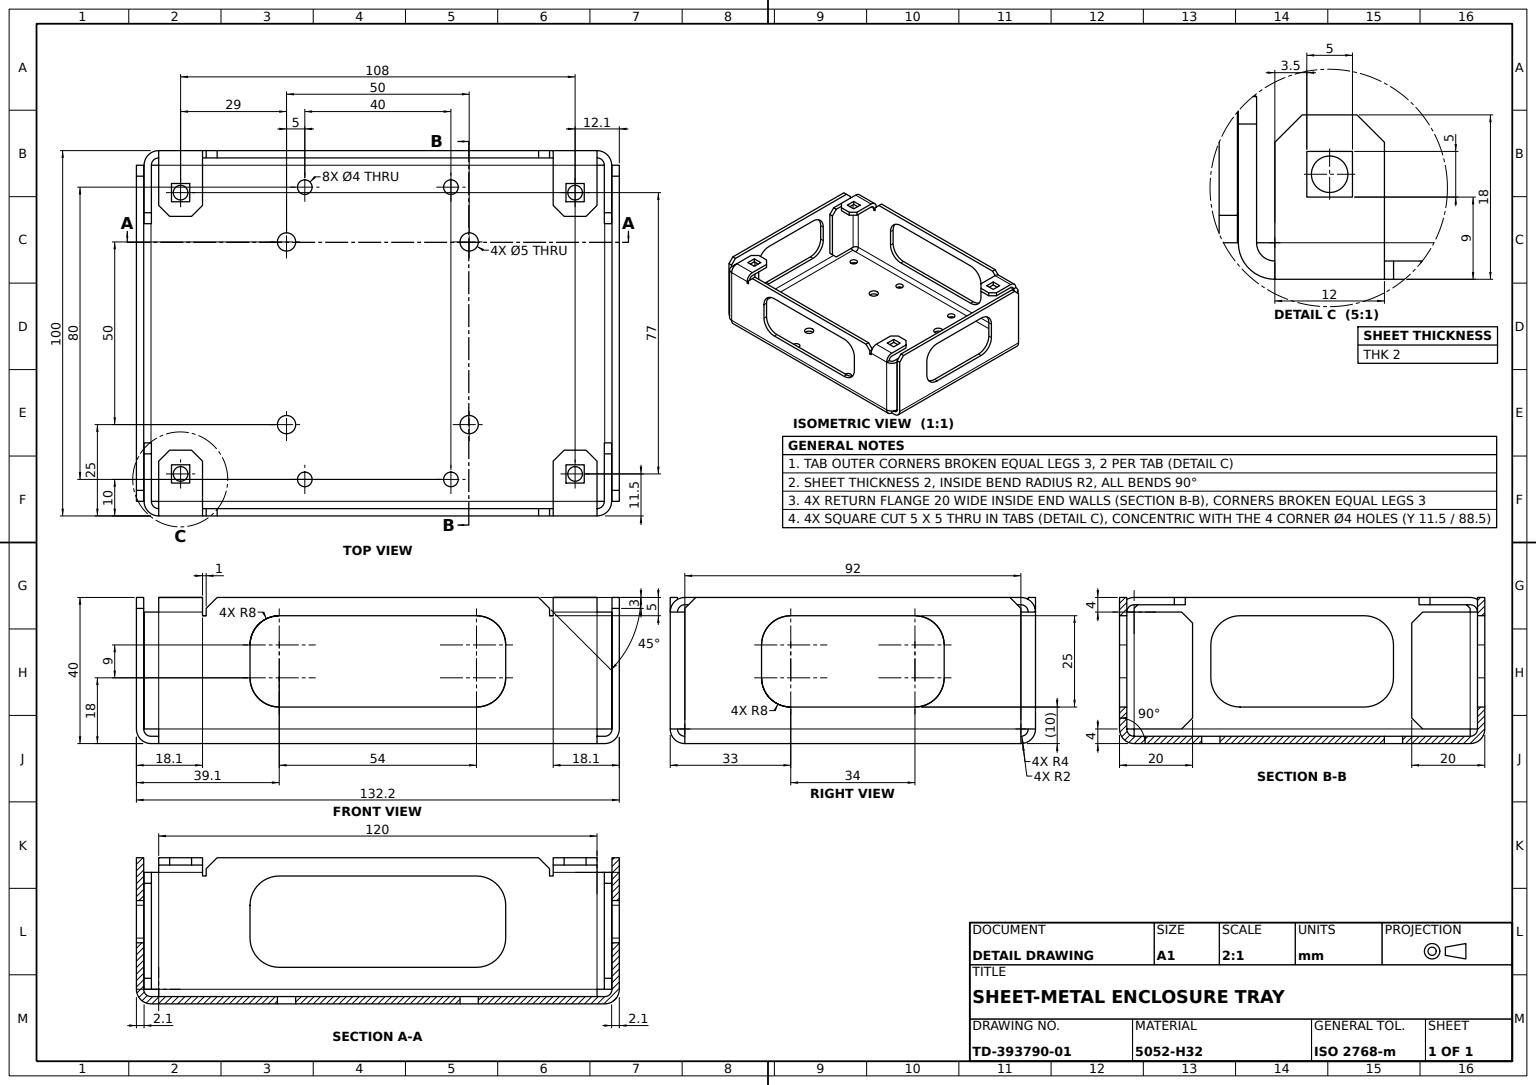
solid
v1 (-27,10,-48)
v2 (27,10,-48)
e1 v1 v2 LINE
v3 (27,10,-50)
e2 v2 v3 LINE
v4 (-27,10,-50)
e3 v4 v3 LINE
e4 v1 v4 LINE
face PLANE(AX(P(-27,10,-48),D(0,1,0),D(0,0,1))) [e1 e2 -e3 -e4]
v5 (-35,27,-48)
v6 (-35,18,-48)
e5 v5 v6 LINE
v7 (-35,18,-50)
e6 v6 v7 LINE
v8 (-35,27,-50)
e7 v8 v7 LINE
e8 v5 v8 LINE
face PLANE(AX(P(-35,18,-48),D(1,0,0),D(0,1,0))) [e5 e6 -e7 -e8]
v9 (47,37,-50)
v10 (47,37,-48)
e9 v9 v10 LINE
v11 (44,40,-50)
e10 v11 v9 LINE
v12 (44,40,-48)
e11 v12 v11 LINE
e12 v10 v12 LINE
face PLANE(AX(P(44,40,-50),D(0.707106781,0.707106781,0),D(0,0,1))) [-e9 -e10 -e11 -e12]
v13 (60,38,46)
v14 (60,36,48)
e13 v13 v14 CIRCLE(AX(P(60,36,46),D(1,0,0),D(0,0,-1)),2)
v15 (60,40,46)
e14 v13 v15 LINE
v16 (60,36,50)
e15 v15 v16 CIRCLE(AX(P(60,36,46),D(1,0,0),D(0,0,-1)),4)
e16 v14 v16 LINE
face PLANE(AX(P(60,36,46),D(-1,0,0),D(0,0,1))) rev [-e13 e14 e15 -e16]
v17 (64.1,18,25)
v18 (66.1,18,25)
e17 v17 v18 LINE
v19 (66.1,10,17)
e18 v18 v19 CIRCLE(AX(P(66.1,18,17),D(1,0,0),D(0,-1,0)),8)
v20 (64.1,10,17)
e19 v20 v19 LINE
e20 v17 v20 CIRCLE(AX(P(64.1,18,17),D(1,0,0),D(0,-1,0)),8)
face CYL(AX(P(64.1,18,17),D(1,0,0),D(0,1,0)),8) rev [e17 e18 -e19 -e20]
v21 (64.1,35,-17)
v22 (66.1,35,-17)
e21 v21 v22 LINE
v23 (64.1,27,-25)
e22 v23 v21 CIRCLE(AX(P(64.1,27,-17),D(1,0,0),D(0,-1,0)),8)
v24 (66.1,27,-25)
e23 v23 v24 LINE
e24 v24 v22 CIRCLE(AX(P(66.1,27,-17),D(1,0,0),D(0,-1,0)),8)
face CYL(AX(P(64.1,27,-17),D(1,0,0),D(0,1,0)),8) rev [-e21 -e22 e23 e24]
v25 (48,38,46)
e25 v25 v13 LINE
v26 (48,38,35)
e26 v26 v25 LINE
v27 (51,38,32)
e27 v26 v27 LINE
v28 (57,38,32)
e28 v28 v27 LINE
v29 (60,38,35)
e29 v28 v29 LINE
e30 v13 v29 LINE
v30 (56.5,38,41)
v31 (56.5,38,36)
e31 v30 v31 LINE
v32 (51.5,38,36)
e32 v31 v32 LINE
v33 (51.5,38,41)
e33 v32 v33 LINE
e34 v33 v30 LINE
face PLANE(AX(P(0,38,0),D(0,-1,0),D(0,0,-1))) [-e25 -e26 e27 -e28 e29 -e30] [e31 e32 e33 e34]
v34 (27,35,-48)
v35 (-27,35,-48)
e35 v34 v35 LINE
v36 (35,27,-48)
e36 v36 v34 CIRCLE(AX(P(27,27,-48),D(0,0,1),D(-1,0,0)),8)
v37 (35,18,-48)
e37 v37 v36 LINE
e38 v2 v37 CIRCLE(AX(P(27,18,-48),D(0,0,1),D(1,0,0)),8)
e39 v6 v1 CIRCLE(AX(P(-27,18,-48),D(0,0,1),D(-1,0,0)),8)
e40 v35 v5 CIRCLE(AX(P(-27,27,-48),D(0,0,1),D(-1,0,0)),8)
v38 (-47,35,-48)
v39 (-47,37,-48)
e41 v38 v39 LINE
v40 (-48,35,-48)
e42 v40 v38 LINE
v41 (-48,36,-48)
e43 v41 v40 LINE
v42 (-60,36,-48)
e44 v42 v41 LINE
v43 (-60,4,-48)
e45 v43 v42 LINE
v44 (60,4,-48)
e46 v44 v43 LINE
v45 (60,36,-48)
e47 v45 v44 LINE
v46 (48,36,-48)
e48 v46 v45 LINE
v47 (48,35,-48)
e49 v47 v46 LINE
v48 (47,35,-48)
e50 v48 v47 LINE
e51 v10 v48 LINE
v49 (-44,40,-48)
e52 v49 v12 LINE
e53 v49 v39 LINE
face PLANE(AX(P(0,0,-48),D(0,0,1),D(0,-1,0))) [-e35 -e36 -e37 -e38 -e1 -e39 -e5 -e40] [-e41 -e42 -e43 -e44 -e45 -e46 -e47 -e48 -e49 -e50 -e51 e12 -e52 e53]
v50 (51.5,40,36)
e54 v32 v50 LINE
v51 (56.5,40,36)
e55 v31 v51 LINE
e56 v51 v50 LINE
face PLANE(AX(P(56.5,38,36),D(0,0,-1),D(0,1,0))) rev [-e54 -e32 e55 e56]
v52 (-47,37,-50)
e57 v39 v52 LINE
v53 (-44,40,-50)
e58 v53 v49 LINE
e59 v52 v53 LINE
face PLANE(AX(P(-47,37,-48),D(-0.707106781,0.707106781,0),D(0,0,1))) [-e57 -e53 -e58 -e59]
v54 (-48,36,-50)
e60 v41 v54 LINE
v55 (-48,35,-50)
e61 v40 v55 LINE
e62 v55 v54 LINE
face PLANE(AX(P(-48,36,-48),D(1,0,0),D(0,0,-1))) [-e60 e43 e61 e62]
v56 (-51.5,38,36)
v57 (-51.5,40,36)
e63 v56 v57 LINE
v58 (-56.5,40,36)
e64 v58 v57 LINE
v59 (-56.5,38,36)
e65 v59 v58 LINE
e66 v59 v56 LINE
face PLANE(AX(P(-56.5,38,36),D(0,0,1),D(0,-1,0))) [e63 -e64 -e65 e66]
v60 (44,40,48)
v61 (47,37,48)
e67 v60 v61 LINE
v62 (44,40,50)
e68 v62 v60 LINE
v63 (47,37,50)
e69 v63 v62 LINE
e70 v61 v63 LINE
face PLANE(AX(P(47,37,48),D(0.707106781,0.707106781,0),D(0,0,-1))) [-e67 -e68 -e69 -e70]
v64 (-62,4,-33)
v65 (-62,4,-46)
e71 v64 v65 LINE
v66 (-62,36,-46)
e72 v66 v65 LINE
v67 (-62,36,-33)
e73 v66 v67 LINE
v68 (-62,33,-30)
e74 v67 v68 LINE
v69 (-62,7,-30)
e75 v68 v69 LINE
e76 v69 v64 LINE
face PLANE(AX(P(-62,0,0),D(1,0,0),D(0,0,-1))) [e71 -e72 e73 e74 e75 e76]
v70 (48,36,-50)
v71 (60,36,-50)
e77 v70 v71 LINE
v72 (48,40,-46)
e78 v72 v70 CIRCLE(AX(P(48,36,-46),D(-1,0,0),D(0,0,1)),4)
v73 (60,40,-46)
e79 v72 v73 LINE
e80 v71 v73 CIRCLE(AX(P(60,36,-46),D(1,0,0),D(0,0,1)),4)
face CYL(AX(P(48,36,-46),D(-1,0,0),D(0,1,0)),4) [-e77 -e78 e79 -e80]
v74 (25,0,-27.5)
v75 (25,2,-27.5)
e81 v74 v75 LINE
v76 (25,0,-22.5)
e82 v76 v74 CIRCLE(AX(P(25,0,-25),D(0,1,0),D(0,0,1)),2.5)
v77 (25,2,-22.5)
e83 v76 v77 LINE
e84 v77 v75 CIRCLE(AX(P(25,2,-25),D(0,1,0),D(0,0,1)),2.5)
face CYL(AX(P(25,0,-25),D(0,1,0),D(0,0,1)),2.5) rev [-e81 -e82 e83 e84]
v78 (-60,4,-50)
v79 (-60,36,-50)
e85 v78 v79 LINE
v80 (-64,4,-46)
e86 v80 v78 CIRCLE(AX(P(-60,4,-46),D(0,-1,0),D(0,0,-1)),4)
v81 (-64,36,-46)
e87 v80 v81 LINE
e88 v79 v81 CIRCLE(AX(P(-60,36,-46),D(0,1,0),D(0,0,-1)),4)
face CYL(AX(P(-60,4,-46),D(0,-1,0),D(-1,0,0)),4) [-e85 -e86 e87 -e88]
v82 (60,2,46)
v83 (60,0,46)
e89 v82 v83 LINE
v84 (62.1,0,46)
e90 v84 v83 LINE
v85 (62.1,2,46)
e91 v85 v84 LINE
e92 v85 v82 LINE
face PLANE(AX(P(62.1,2,46),D(0,0,-1),D(0,-1,0))) rev [e89 -e90 -e91 e92]
v86 (62,7,-30)
v87 (62,33,-30)
e93 v86 v87 LINE
v88 (64,7,-30)
e94 v86 v88 LINE
v89 (64,33,-30)
e95 v88 v89 LINE
e96 v89 v87 LINE
face PLANE(AX(P(64,4,-30),D(0,0,1),D(1,0,0))) [-e93 e94 e95 e96]
v90 (64.1,18,-25)
e97 v90 v23 LINE
v91 (64.1,35,17)
e98 v21 v91 LINE
v92 (64.1,27,25)
e99 v91 v92 CIRCLE(AX(P(64.1,27,17),D(1,0,0),D(0,-1,0)),8)
e100 v92 v17 LINE
v93 (64.1,10,-17)
e101 v20 v93 LINE
e102 v93 v90 CIRCLE(AX(P(64.1,18,-17),D(1,0,0),D(0,1,0)),8)
v94 (64.1,4,46)
v95 (64.1,4,-46)
e103 v94 v95 LINE
v96 (64.1,37,46)
e104 v96 v94 LINE
v97 (64.1,40,43)
e105 v96 v97 LINE
v98 (64.1,40,-43)
e106 v98 v97 LINE
v99 (64.1,37,-46)
e107 v98 v99 LINE
e108 v95 v99 LINE
face PLANE(AX(P(64.1,0,0),D(-1,0,0),D(0,-1,0))) [e97 e22 e98 e99 e100 e20 e101 e102] [-e103 -e104 e105 -e106 e107 -e108]
v100 (54,0,36.5)
v101 (54,2,36.5)
e109 v100 v101 LINE
v102 (54,2,40.5)
e110 v101 v102 CIRCLE(AX(P(54,2,38.5),D(0,1,0),D(0,0,1)),2)
v103 (54,0,40.5)
e111 v103 v102 LINE
e112 v100 v103 CIRCLE(AX(P(54,0,38.5),D(0,1,0),D(0,0,1)),2)
face CYL(AX(P(54,0,38.5),D(0,1,0),D(0,0,1)),2) rev [e109 e110 -e111 -e112]
v104 (-51.5,40,41)
v105 (-56.5,40,41)
e113 v104 v105 LINE
v106 (-51.5,38,41)
e114 v106 v104 LINE
v107 (-56.5,38,41)
e115 v106 v107 LINE
e116 v107 v105 LINE
face PLANE(AX(P(-56.5,38,41),D(0,0,-1),D(0,1,0))) [-e113 -e114 e115 e116]
v108 (47,35,50)
e117 v63 v108 LINE
v109 (47,35,48)
e118 v109 v108 LINE
e119 v109 v61 LINE
face PLANE(AX(P(47,35,48),D(1,0,0),D(0,0,-1))) [e117 -e118 e119 e70]
v110 (-64.1,35,17)
v111 (-64.1,27,25)
e120 v110 v111 CIRCLE(AX(P(-64.1,27,17),D(1,0,0),D(0,-1,0)),8)
v112 (-66.1,27,25)
e121 v111 v112 LINE
v113 (-66.1,35,17)
e122 v113 v112 CIRCLE(AX(P(-66.1,27,17),D(1,0,0),D(0,-1,0)),8)
e123 v110 v113 LINE
face CYL(AX(P(-64.1,27,17),D(-1,0,0),D(0,-1,0)),8) rev [e120 e121 -e122 -e123]
v114 (-35,18,48)
v115 (-35,18,50)
e124 v114 v115 LINE
v116 (-27,10,50)
e125 v115 v116 CIRCLE(AX(P(-27,18,50),D(0,0,1),D(-1,0,0)),8)
v117 (-27,10,48)
e126 v117 v116 LINE
e127 v114 v117 CIRCLE(AX(P(-27,18,48),D(0,0,1),D(-1,0,0)),8)
face CYL(AX(P(-27,18,48),D(0,0,1),D(1,0,0)),8) rev [e124 e125 -e126 -e127]
v118 (-54,2,-40.5)
v119 (-54,2,-36.5)
e128 v118 v119 CIRCLE(AX(P(-54,2,-38.5),D(0,1,0),D(0,0,1)),2)
v120 (-54,0,-36.5)
e129 v120 v119 LINE
v121 (-54,0,-40.5)
e130 v121 v120 CIRCLE(AX(P(-54,0,-38.5),D(0,1,0),D(0,0,1)),2)
e131 v121 v118 LINE
face CYL(AX(P(-54,0,-38.5),D(0,1,0),D(0,0,1)),2) rev [e128 -e129 -e130 e131]
v122 (-64.1,18,-25)
v123 (-64.1,27,-25)
e132 v122 v123 LINE
v124 (-66.1,27,-25)
e133 v123 v124 LINE
v125 (-66.1,18,-25)
e134 v125 v124 LINE
e135 v122 v125 LINE
face PLANE(AX(P(-64.1,18,-25),D(0,0,1),D(1,0,0))) [e132 e133 -e134 -e135]
v126 (35,27,-50)
v127 (27,35,-50)
e136 v126 v127 CIRCLE(AX(P(27,27,-50),D(0,0,1),D(-1,0,0)),8)
v128 (-27,35,-50)
e137 v127 v128 LINE
e138 v128 v8 CIRCLE(AX(P(-27,27,-50),D(0,0,1),D(-1,0,0)),8)
e139 v7 v4 CIRCLE(AX(P(-27,18,-50),D(0,0,1),D(-1,0,0)),8)
v129 (35,18,-50)
e140 v3 v129 CIRCLE(AX(P(27,18,-50),D(0,0,1),D(1,0,0)),8)
e141 v129 v126 LINE
v130 (-47,35,-50)
e142 v52 v130 LINE
e143 v53 v11 LINE
v131 (47,35,-50)
e144 v131 v9 LINE
v132 (48,35,-50)
e145 v132 v131 LINE
e146 v70 v132 LINE
v133 (60,4,-50)
e147 v71 v133 LINE
e148 v78 v133 LINE
e149 v79 v54 LINE
e150 v130 v55 LINE
face PLANE(AX(P(0,0,-50),D(0,0,1),D(0,-1,0))) rev [e136 e137 e138 e7 e139 e3 e140 e141] [-e142 e59 e143 e10 -e144 -e145 -e146 e77 e147 -e148 e85 e149 -e62 -e150]
face PLANE(AX(P(60,40,-50),D(0,-1,0),D(0,0,-1))) rev [e52 e11 -e143 e58]
v134 (66.1,35,17)
e151 v22 v134 LINE
e152 v91 v134 LINE
face PLANE(AX(P(64.1,35,17),D(0,1,0),D(-1,0,0))) rev [e21 e151 -e152 -e98]
v135 (-44,40,50)
e153 v62 v135 LINE
v136 (-47,37,50)
e154 v135 v136 LINE
v137 (-47,35,50)
e155 v137 v136 LINE
v138 (-48,35,50)
e156 v138 v137 LINE
v139 (-48,36,50)
e157 v139 v138 LINE
v140 (-60,36,50)
e158 v139 v140 LINE
v141 (-60,4,50)
e159 v140 v141 LINE
v142 (60,4,50)
e160 v142 v141 LINE
e161 v142 v16 LINE
v143 (48,36,50)
e162 v16 v143 LINE
v144 (48,35,50)
e163 v144 v143 LINE
e164 v108 v144 LINE
v145 (35,18,50)
v146 (35,27,50)
e165 v145 v146 LINE
v147 (27,10,50)
e166 v147 v145 CIRCLE(AX(P(27,18,50),D(0,0,1),D(1,0,0)),8)
e167 v116 v147 LINE
v148 (-35,27,50)
e168 v148 v115 LINE
v149 (-27,35,50)
e169 v149 v148 CIRCLE(AX(P(-27,27,50),D(0,0,1),D(-1,0,0)),8)
v150 (27,35,50)
e170 v150 v149 LINE
e171 v146 v150 CIRCLE(AX(P(27,27,50),D(0,0,1),D(-1,0,0)),8)
face PLANE(AX(P(0,0,50),D(0,0,-1),D(-1,0,0))) rev [e69 e153 e154 -e155 -e156 -e157 e158 e159 -e160 e161 e162 -e163 -e164 -e117] [-e165 -e166 -e167 -e125 -e168 -e169 -e170 -e171]
v151 (-48,38,-46)
v152 (-48,40,-46)
e172 v151 v152 LINE
v153 (-48,40,-35)
e173 v153 v152 LINE
v154 (-48,38,-35)
e174 v153 v154 LINE
e175 v154 v151 LINE
face PLANE(AX(P(-48,40,-48),D(-1,0,0),D(0,0,1))) rev [e172 -e173 e174 e175]
v155 (48,36,48)
e176 v14 v155 LINE
e177 v155 v25 CIRCLE(AX(P(48,36,46),D(-1,0,0),D(0,0,-1)),2)
face CYL(AX(P(60,36,46),D(1,0,0),D(0,1,0)),2) rev [e176 e177 e25 e13]
v156 (54,0,-36.5)
v157 (54,0,-40.5)
e178 v156 v157 CIRCLE(AX(P(54,0,-38.5),D(0,1,0),D(0,0,1)),2)
v158 (54,2,-36.5)
e179 v156 v158 LINE
v159 (54,2,-40.5)
e180 v158 v159 CIRCLE(AX(P(54,2,-38.5),D(0,1,0),D(0,0,1)),2)
e181 v157 v159 LINE
face CYL(AX(P(54,0,-38.5),D(0,1,0),D(0,0,1)),2) rev [-e178 e179 e180 -e181]
v160 (-64,4,-33)
e182 v160 v80 LINE
e183 v65 v80 LINE
e184 v64 v160 LINE
face PLANE(AX(P(-64,4,-30),D(0,-1,0),D(0,0,-1))) [e182 -e183 -e71 e184]
v161 (-60,40,-46)
e185 v161 v79 CIRCLE(AX(P(-60,36,-46),D(-1,0,0),D(0,0,1)),4)
e186 v161 v152 LINE
e187 v54 v152 CIRCLE(AX(P(-48,36,-46),D(1,0,0),D(0,0,1)),4)
face CYL(AX(P(-60,36,-46),D(-1,0,0),D(0,1,0)),4) [-e185 e186 -e187 -e149]
v162 (-57,40,-32)
v163 (-51,40,-32)
e188 v162 v163 LINE
e189 v163 v153 LINE
v164 (-60,40,-35)
e190 v161 v164 LINE
e191 v164 v162 LINE
v165 (-51.5,40,-41)
v166 (-56.5,40,-41)
e192 v165 v166 LINE
v167 (-51.5,40,-36)
e193 v167 v165 LINE
v168 (-56.5,40,-36)
e194 v168 v167 LINE
e195 v166 v168 LINE
face PLANE(AX(P(0,40,0),D(0,-1,0),D(0,0,1))) rev [e188 e189 e173 -e186 e190 e191] [-e192 -e193 -e194 -e195]
v169 (60,40,-35)
v170 (60,38,-35)
e196 v169 v170 LINE
v171 (57,40,-32)
e197 v171 v169 LINE
v172 (57,38,-32)
e198 v172 v171 LINE
e199 v170 v172 LINE
face PLANE(AX(P(60,40,-35),D(-0.707106781,0,-0.707106781),D(0,-1,0))) rev [-e196 -e197 -e198 -e199]
v173 (57,40,32)
e200 v173 v28 LINE
v174 (51,40,32)
e201 v27 v174 LINE
e202 v173 v174 LINE
face PLANE(AX(P(48,40,32),D(0,0,1),D(0,-1,0))) rev [e200 e28 e201 -e202]
v175 (-48,40,35)
v176 (-48,40,46)
e203 v175 v176 LINE
v177 (-48,38,46)
e204 v177 v176 LINE
v178 (-48,38,35)
e205 v178 v177 LINE
e206 v178 v175 LINE
face PLANE(AX(P(-48,40,48),D(1,0,0),D(0,0,-1))) [e203 -e204 -e205 e206]
v179 (20,0,38)
v180 (20,2,38)
e207 v179 v180 LINE
v181 (20,0,42)
e208 v181 v179 CIRCLE(AX(P(20,0,40),D(0,1,0),D(0,0,1)),2)
v182 (20,2,42)
e209 v181 v182 LINE
e210 v182 v180 CIRCLE(AX(P(20,2,40),D(0,1,0),D(0,0,1)),2)
face CYL(AX(P(20,0,40),D(0,1,0),D(0,0,1)),2) rev [-e207 -e208 e209 e210]
v183 (-64,4,46)
e211 v141 v183 CIRCLE(AX(P(-60,4,46),D(0,-1,0),D(0,0,1)),4)
v184 (-64,36,46)
e212 v184 v140 CIRCLE(AX(P(-60,36,46),D(0,1,0),D(0,0,1)),4)
e213 v184 v183 LINE
face CYL(AX(P(-60,36,46),D(0,1,0),D(-1,0,0)),4) [-e211 -e159 -e212 e213]
v185 (-56.5,38,-41)
e214 v185 v166 LINE
v186 (-51.5,38,-41)
e215 v186 v185 LINE
e216 v186 v165 LINE
face PLANE(AX(P(-56.5,38,-41),D(0,0,-1),D(0,1,0))) rev [e192 -e214 -e215 e216]
v187 (-64,7,-30)
e217 v187 v69 LINE
e218 v160 v187 LINE
face PLANE(AX(P(-64,7,-30),D(0,0.707106781,-0.707106781),D(1,0,0))) rev [-e217 -e218 -e184 -e76]
v188 (62.1,2,-46)
v189 (62.1,0,-46)
e219 v188 v189 LINE
v190 (60,0,-46)
e220 v189 v190 LINE
v191 (60,2,-46)
e221 v191 v190 LINE
e222 v188 v191 LINE
face PLANE(AX(P(62.1,2,-46),D(0,0,-1),D(0,-1,0))) [e219 e220 -e221 -e222]
v192 (60,40,35)
e223 v29 v192 LINE
e224 v192 v173 LINE
face PLANE(AX(P(57,40,32),D(-0.707106781,0,0.707106781),D(0,-1,0))) rev [-e223 -e29 -e200 -e224]
v193 (-47,35,48)
e225 v193 v137 LINE
v194 (-47,37,48)
e226 v136 v194 LINE
e227 v194 v193 LINE
face PLANE(AX(P(-47,40,48),D(-1,0,0),D(0,0,1))) [e225 e155 e226 e227]
v195 (-57,38,-32)
v196 (-60,38,-35)
e228 v195 v196 LINE
e229 v162 v195 LINE
e230 v196 v164 LINE
face PLANE(AX(P(-57,40,-32),D(0.707106781,0,-0.707106781),D(0,-1,0))) rev [-e228 -e229 -e191 -e230]
v197 (62,36,-33)
v198 (62,36,-46)
e231 v197 v198 LINE
v199 (64,36,-33)
e232 v197 v199 LINE
v200 (64,36,-46)
e233 v199 v200 LINE
e234 v198 v200 LINE
face PLANE(AX(P(64,36,-30),D(0,1,0),D(0,0,1))) [-e231 e232 e233 -e234]
v201 (-48,35,48)
e235 v201 v138 LINE
v202 (-48,36,48)
e236 v201 v202 LINE
e237 v202 v139 LINE
face PLANE(AX(P(-48,35,48),D(1,0,0),D(0,0,-1))) [e157 -e235 e236 e237]
v203 (66.1,40,43)
e238 v97 v203 LINE
v204 (66.1,37,46)
e239 v204 v96 LINE
e240 v203 v204 LINE
face PLANE(AX(P(66.1,37,46),D(0,-0.707106781,-0.707106781),D(-1,0,0))) rev [-e238 -e105 -e239 -e240]
v205 (56.5,40,41)
e241 v30 v205 LINE
e242 v205 v51 LINE
face PLANE(AX(P(56.5,38,36),D(1,0,0),D(0,0,-1))) rev [e241 e242 -e55 -e31]
e243 v66 v81 LINE
v206 (-64,36,-33)
e244 v81 v206 LINE
e245 v206 v67 LINE
face PLANE(AX(P(-64,36,-48),D(0,1,0),D(0,0,1))) [-e73 e243 e244 e245]
v207 (-51,38,-32)
e246 v195 v207 LINE
e247 v207 v163 LINE
face PLANE(AX(P(-48,40,-32),D(0,0,-1),D(0,1,0))) rev [e246 e247 -e188 e229]
v208 (-60,40,46)
e248 v176 v208 LINE
e249 v140 v208 CIRCLE(AX(P(-60,36,46),D(-1,0,0),D(0,0,-1)),4)
e250 v176 v139 CIRCLE(AX(P(-48,36,46),D(1,0,0),D(0,0,-1)),4)
face CYL(AX(P(-48,36,46),D(1,0,0),D(0,1,0)),4) [e248 -e249 -e158 -e250]
v209 (-51.5,38,-36)
e251 v209 v186 LINE
e252 v209 v167 LINE
face PLANE(AX(P(-51.5,38,-36),D(1,0,0),D(0,0,-1))) rev [-e216 -e251 e252 e193]
v210 (-60,38,46)
e253 v210 v208 LINE
v211 (-60,36,48)
e254 v211 v210 CIRCLE(AX(P(-60,36,46),D(-1,0,0),D(0,0,-1)),2)
e255 v211 v140 LINE
face PLANE(AX(P(-60,36,46),D(-1,0,0),D(0,0,1))) [e249 -e253 -e254 e255]
v212 (-54,2,36.5)
v213 (-54,2,40.5)
e256 v212 v213 CIRCLE(AX(P(-54,2,38.5),D(0,1,0),D(0,0,1)),2)
v214 (-54,0,40.5)
e257 v214 v213 LINE
v215 (-54,0,36.5)
e258 v215 v214 CIRCLE(AX(P(-54,0,38.5),D(0,1,0),D(0,0,1)),2)
e259 v215 v212 LINE
face CYL(AX(P(-54,0,38.5),D(0,1,0),D(0,0,1)),2) rev [e256 -e257 -e258 e259]
v216 (25,0,27.5)
v217 (25,0,22.5)
e260 v216 v217 CIRCLE(AX(P(25,0,25),D(0,1,0),D(0,0,1)),2.5)
v218 (25,2,27.5)
e261 v216 v218 LINE
v219 (25,2,22.5)
e262 v218 v219 CIRCLE(AX(P(25,2,25),D(0,1,0),D(0,0,1)),2.5)
e263 v217 v219 LINE
face CYL(AX(P(25,0,25),D(0,1,0),D(0,0,1)),2.5) rev [-e260 e261 e262 -e263]
v220 (66.1,4,-46)
v221 (66.1,4,46)
e264 v220 v221 LINE
e265 v84 v221 CIRCLE(AX(P(62.1,4,46),D(0,0,1),D(-1,0,0)),4)
e266 v189 v84 LINE
e267 v220 v189 CIRCLE(AX(P(62.1,4,-46),D(0,0,-1),D(-1,0,0)),4)
face CYL(AX(P(62.1,4,-46),D(0,0,-1),D(1,0,0)),4) [e264 -e265 -e266 -e267]
v222 (62,33,30)
v223 (62,7,30)
e268 v222 v223 LINE
v224 (62,4,33)
e269 v223 v224 LINE
v225 (62,4,46)
e270 v224 v225 LINE
v226 (62,36,46)
e271 v226 v225 LINE
v227 (62,36,33)
e272 v226 v227 LINE
e273 v227 v222 LINE
face PLANE(AX(P(62,0,0),D(1,0,0),D(0,0,-1))) rev [e268 e269 e270 -e271 e272 e273]
v228 (-64.1,4,46)
v229 (-66.1,4,46)
e274 v228 v229 LINE
v230 (-62.1,0,46)
e275 v229 v230 CIRCLE(AX(P(-62.1,4,46),D(0,0,1),D(1,0,0)),4)
v231 (-62.1,2,46)
e276 v231 v230 LINE
e277 v228 v231 CIRCLE(AX(P(-62.1,4,46),D(0,0,1),D(1,0,0)),2)
face PLANE(AX(P(-62.1,4,46),D(0,0,-1),D(-1,0,0))) rev [e274 e275 -e276 -e277]
e278 v198 v45 CIRCLE(AX(P(60,36,-46),D(0,1,0),D(0,0,1)),2)
e279 v200 v71 CIRCLE(AX(P(60,36,-46),D(0,1,0),D(0,0,1)),4)
e280 v45 v71 LINE
face PLANE(AX(P(60,36,-46),D(0,-1,0),D(0,0,-1))) rev [-e278 e234 e279 -e280]
e281 v36 v126 LINE
e282 v34 v127 LINE
face CYL(AX(P(27,27,-48),D(0,0,-1),D(-1,0,0)),8) rev [-e281 e36 e282 -e136]
v232 (64,4,-33)
e283 v88 v232 LINE
v233 (64,4,-46)
e284 v233 v232 LINE
e285 v200 v233 LINE
e286 v199 v89 LINE
face PLANE(AX(P(64,0,0),D(-1,0,0),D(0,0,1))) rev [-e95 e283 -e284 -e285 -e233 e286]
v234 (66.1,40,-43)
e287 v234 v98 LINE
v235 (66.1,37,-46)
e288 v235 v234 LINE
e289 v99 v235 LINE
face PLANE(AX(P(66.1,40,-43),D(0,-0.707106781,0.707106781),D(-1,0,0))) rev [-e287 -e288 -e289 -e107]
v236 (-60,4,48)
v237 (-62,4,46)
e290 v236 v237 CIRCLE(AX(P(-60,4,46),D(0,-1,0),D(0,0,1)),2)
v238 (-62,36,46)
e291 v237 v238 LINE
e292 v238 v211 CIRCLE(AX(P(-60,36,46),D(0,1,0),D(0,0,1)),2)
e293 v211 v236 LINE
face CYL(AX(P(-60,36,46),D(0,1,0),D(-1,0,0)),2) rev [e290 e291 e292 e293]
e294 v35 v128 LINE
face CYL(AX(P(-27,27,-48),D(0,0,-1),D(-1,0,0)),8) rev [e8 -e138 -e294 e40]
e295 v213 v212 CIRCLE(AX(P(-54,2,38.5),D(0,1,0),D(0,0,1)),2)
e296 v214 v215 CIRCLE(AX(P(-54,0,38.5),D(0,1,0),D(0,0,1)),2)
face CYL(AX(P(-54,0,38.5),D(0,1,0),D(0,0,1)),2) rev [e295 -e259 -e296 e257]
v239 (48,40,35)
e297 v239 v26 LINE
e298 v174 v239 LINE
face PLANE(AX(P(48,40,35),D(0.707106781,0,0.707106781),D(0,-1,0))) rev [-e201 -e27 -e297 -e298]
v240 (-64.1,4,-46)
v241 (-66.1,4,-46)
e299 v240 v241 LINE
v242 (-66.1,37,-46)
e300 v242 v241 LINE
v243 (-64.1,37,-46)
e301 v242 v243 LINE
e302 v243 v240 LINE
face PLANE(AX(P(-66.1,2,-46),D(0,0,1),D(1,0,0))) rev [e299 -e300 e301 e302]
v244 (-51,40,32)
e303 v175 v244 LINE
v245 (-57,40,32)
e304 v245 v244 LINE
v246 (-60,40,35)
e305 v245 v246 LINE
e306 v208 v246 LINE
e307 v105 v58 LINE
e308 v57 v104 LINE
face PLANE(AX(P(0,40,0),D(0,-1,0),D(0,0,-1))) rev [e303 -e304 e305 -e306 -e248 -e203] [e307 e64 e308 e113]
v247 (62,4,-46)
e309 v44 v247 CIRCLE(AX(P(60,4,-46),D(0,-1,0),D(0,0,1)),2)
e310 v44 v133 LINE
e311 v133 v233 CIRCLE(AX(P(60,4,-46),D(0,-1,0),D(0,0,1)),4)
e312 v247 v233 LINE
face PLANE(AX(P(60,4,-46),D(0,-1,0),D(0,0,-1))) [-e309 e310 e311 -e312]
v248 (48,40,-35)
e313 v248 v72 LINE
v249 (51,40,-32)
e314 v248 v249 LINE
e315 v171 v249 LINE
e316 v73 v169 LINE
v250 (56.5,40,-36)
v251 (51.5,40,-36)
e317 v250 v251 LINE
v252 (51.5,40,-41)
e318 v251 v252 LINE
v253 (56.5,40,-41)
e319 v252 v253 LINE
e320 v253 v250 LINE
face PLANE(AX(P(0,40,0),D(0,-1,0),D(0,0,1))) rev [-e79 -e313 e314 -e315 e197 -e316] [e317 e318 e319 e320]
e321 v217 v216 CIRCLE(AX(P(25,0,25),D(0,1,0),D(0,0,1)),2.5)
e322 v219 v218 CIRCLE(AX(P(25,2,25),D(0,1,0),D(0,0,1)),2.5)
face CYL(AX(P(25,0,25),D(0,1,0),D(0,0,1)),2.5) rev [-e321 e263 e322 -e261]
e323 v37 v129 LINE
face CYL(AX(P(27,18,-48),D(0,0,-1),D(-1,0,0)),8) rev [-e140 -e2 e38 e323]
v254 (-56.5,38,-36)
e324 v254 v209 LINE
e325 v254 v168 LINE
face PLANE(AX(P(-56.5,38,-36),D(0,0,1),D(0,-1,0))) rev [e194 -e252 -e324 e325]
v255 (66.1,18,-25)
e326 v90 v255 LINE
e327 v255 v24 LINE
face PLANE(AX(P(64.1,18,-25),D(0,0,-1),D(-1,0,0))) rev [-e97 e326 e327 -e23]
e328 v220 v235 LINE
e329 v95 v220 LINE
face PLANE(AX(P(66.1,40,-46),D(0,0,1),D(1,0,0))) rev [-e328 -e329 e108 e289]
e330 v15 v192 LINE
v256 (48,40,46)
e331 v239 v256 LINE
e332 v15 v256 LINE
v257 (51.5,40,41)
e333 v50 v257 LINE
e334 v257 v205 LINE
face PLANE(AX(P(0,40,0),D(0,-1,0),D(0,0,-1))) rev [e330 e224 e202 e298 e331 -e332] [-e333 -e56 -e242 -e334]
e335 v56 v106 LINE
e336 v107 v59 LINE
e337 v210 v177 LINE
v258 (-60,38,35)
e338 v210 v258 LINE
v259 (-57,38,32)
e339 v258 v259 LINE
v260 (-51,38,32)
e340 v259 v260 LINE
e341 v260 v178 LINE
face PLANE(AX(P(0,38,0),D(0,-1,0),D(0,0,-1))) [-e335 -e66 -e336 -e115] [-e337 e338 e339 e340 e341 e205]
v261 (64,33,30)
v262 (64,36,33)
e342 v261 v262 LINE
v263 (64,36,46)
e343 v263 v262 LINE
v264 (64,4,46)
e344 v263 v264 LINE
v265 (64,4,33)
e345 v265 v264 LINE
v266 (64,7,30)
e346 v265 v266 LINE
e347 v261 v266 LINE
face PLANE(AX(P(64,0,0),D(1,0,0),D(0,0,-1))) [e342 -e343 e344 -e345 e346 -e347]
e348 v225 v264 LINE
e349 v264 v142 CIRCLE(AX(P(60,4,46),D(0,-1,0),D(0,0,-1)),4)
v267 (60,4,48)
e350 v267 v142 LINE
e351 v225 v267 CIRCLE(AX(P(60,4,46),D(0,-1,0),D(0,0,-1)),2)
face PLANE(AX(P(60,4,46),D(0,1,0),D(0,0,1))) rev [e348 e349 -e350 -e351]
e352 v240 v228 LINE
v268 (-64.1,40,-43)
e353 v243 v268 LINE
v269 (-64.1,40,43)
e354 v269 v268 LINE
v270 (-64.1,37,46)
e355 v269 v270 LINE
e356 v228 v270 LINE
v271 (-64.1,18,25)
v272 (-64.1,10,17)
e357 v271 v272 CIRCLE(AX(P(-64.1,18,17),D(1,0,0),D(0,-1,0)),8)
e358 v111 v271 LINE
v273 (-64.1,35,-17)
e359 v273 v110 LINE
e360 v123 v273 CIRCLE(AX(P(-64.1,27,-17),D(1,0,0),D(0,-1,0)),8)
v274 (-64.1,10,-17)
e361 v274 v122 CIRCLE(AX(P(-64.1,18,-17),D(1,0,0),D(0,1,0)),8)
e362 v272 v274 LINE
face PLANE(AX(P(-64.1,0,0),D(1,0,0),D(0,1,0))) [-e352 -e302 e353 -e354 e355 -e356] [-e357 -e358 -e120 -e359 -e360 -e132 -e361 -e362]
v275 (27,35,48)
e363 v275 v150 LINE
v276 (35,27,48)
e364 v276 v275 CIRCLE(AX(P(27,27,48),D(0,0,1),D(-1,0,0)),8)
e365 v276 v146 LINE
face CYL(AX(P(27,27,48),D(0,0,1),D(1,0,0)),8) rev [-e363 -e364 e365 e171]
e366 v238 v184 LINE
face PLANE(AX(P(-60,36,46),D(0,-1,0),D(0,0,-1))) rev [-e255 -e292 e366 e212]
e367 v204 v221 LINE
e368 v94 v221 LINE
face PLANE(AX(P(66.1,2,46),D(0,0,-1),D(-1,0,0))) rev [-e367 e239 e104 e368]
v277 (-20,2,42)
v278 (-20,2,38)
e369 v277 v278 CIRCLE(AX(P(-20,2,40),D(0,1,0),D(0,0,1)),2)
v279 (-20,0,38)
e370 v279 v278 LINE
v280 (-20,0,42)
e371 v280 v279 CIRCLE(AX(P(-20,0,40),D(0,1,0),D(0,0,1)),2)
e372 v280 v277 LINE
face CYL(AX(P(-20,0,40),D(0,1,0),D(0,0,1)),2) rev [e369 -e370 -e371 e372]
v281 (-60,38,-46)
e373 v281 v161 LINE
e374 v281 v196 LINE
face PLANE(AX(P(-60,40,-32),D(1,0,0),D(0,0,-1))) rev [-e190 -e373 e374 e230]
e375 v244 v260 LINE
e376 v259 v245 LINE
face PLANE(AX(P(-48,40,32),D(0,0,-1),D(0,1,0))) [e304 e375 -e340 e376]
e377 v48 v131 LINE
face PLANE(AX(P(47,40,-48),D(1,0,0),D(0,0,-1))) [e144 e9 e51 e377]
v282 (48,38,-46)
e378 v282 v72 LINE
v283 (48,38,-35)
e379 v283 v282 LINE
e380 v283 v248 LINE
face PLANE(AX(P(48,40,-48),D(-1,0,0),D(0,0,1))) [e313 -e378 -e379 e380]
v284 (-62,4,33)
e381 v237 v284 LINE
e382 v237 v183 LINE
v285 (-64,4,33)
e383 v183 v285 LINE
e384 v285 v284 LINE
face PLANE(AX(P(-64,4,48),D(0,-1,0),D(0,0,-1))) [-e381 e382 e383 e384]
e385 v119 v118 CIRCLE(AX(P(-54,2,-38.5),D(0,1,0),D(0,0,1)),2)
e386 v120 v121 CIRCLE(AX(P(-54,0,-38.5),D(0,1,0),D(0,0,1)),2)
face CYL(AX(P(-54,0,-38.5),D(0,1,0),D(0,0,1)),2) rev [e129 e385 -e131 -e386]
v286 (62,4,-33)
e387 v286 v86 LINE
e388 v232 v286 LINE
face PLANE(AX(P(64,4,-33),D(0,0.707106781,-0.707106781),D(-1,0,0))) rev [-e94 -e387 -e388 -e283]
e389 v267 v82 CIRCLE(AX(P(60,4,46),D(1,0,0),D(0,0,-1)),2)
e390 v142 v83 CIRCLE(AX(P(60,4,46),D(1,0,0),D(0,0,-1)),4)
face PLANE(AX(P(60,4,46),D(-1,0,0),D(0,0,1))) rev [-e89 -e389 e350 e390]
v287 (-44,40,48)
e391 v287 v135 LINE
e392 v194 v287 LINE
face PLANE(AX(P(-44,40,50),D(-0.707106781,0.707106781,0),D(0,0,-1))) [-e154 -e391 -e392 -e226]
e393 v247 v198 LINE
e394 v247 v286 LINE
e395 v87 v197 LINE
face PLANE(AX(P(62,0,0),D(-1,0,0),D(0,0,1))) [e231 -e393 e394 e387 e93 e395]
face PLANE(AX(P(60,40,32),D(-1,0,0),D(0,0,1))) rev [-e14 e30 e223 -e330]
e396 v25 v256 LINE
face PLANE(AX(P(48,40,48),D(1,0,0),D(0,0,-1))) rev [e396 -e331 e297 e26]
v288 (51.5,38,-36)
v289 (51.5,38,-41)
e397 v288 v289 LINE
e398 v289 v252 LINE
e399 v288 v251 LINE
face PLANE(AX(P(51.5,38,-36),D(1,0,0),D(0,0,-1))) [e397 e398 -e318 -e399]
v290 (66.1,10,-17)
e400 v93 v290 LINE
e401 v290 v255 CIRCLE(AX(P(66.1,18,-17),D(1,0,0),D(0,1,0)),8)
face CYL(AX(P(64.1,18,-17),D(1,0,0),D(0,1,0)),8) rev [e400 e401 -e326 -e102]
v291 (-25,0,-22.5)
v292 (-25,0,-27.5)
e402 v291 v292 CIRCLE(AX(P(-25,0,-25),D(0,1,0),D(0,0,1)),2.5)
v293 (-25,2,-22.5)
e403 v291 v293 LINE
v294 (-25,2,-27.5)
e404 v293 v294 CIRCLE(AX(P(-25,2,-25),D(0,1,0),D(0,0,1)),2.5)
e405 v292 v294 LINE
face CYL(AX(P(-25,0,-25),D(0,1,0),D(0,0,1)),2.5) rev [-e402 e403 e404 -e405]
e406 v226 v263 LINE
e407 v14 v226 CIRCLE(AX(P(60,36,46),D(0,1,0),D(0,0,-1)),2)
e408 v16 v263 CIRCLE(AX(P(60,36,46),D(0,1,0),D(0,0,-1)),4)
face PLANE(AX(P(60,36,46),D(0,1,0),D(0,0,1))) [-e406 -e407 e16 e408]
e409 v95 v188 CIRCLE(AX(P(62.1,4,-46),D(0,0,-1),D(-1,0,0)),2)
face PLANE(AX(P(62.1,4,-46),D(0,0,1),D(1,0,0))) rev [e329 e267 -e219 -e409]
v295 (-64,33,-30)
e410 v68 v295 LINE
e411 v295 v187 LINE
face PLANE(AX(P(-64,36,-30),D(0,0,1),D(1,0,0))) [e410 e411 e217 -e75]
e412 v279 v280 CIRCLE(AX(P(-20,0,40),D(0,1,0),D(0,0,1)),2)
e413 v278 v277 CIRCLE(AX(P(-20,2,40),D(0,1,0),D(0,0,1)),2)
face CYL(AX(P(-20,0,40),D(0,1,0),D(0,0,1)),2) rev [-e372 -e412 e370 e413]
face CYL(AX(P(60,4,46),D(0,-1,0),D(1,0,0)),4) [-e349 -e344 -e408 -e161]
v296 (56.5,38,-41)
e414 v289 v296 LINE
e415 v296 v253 LINE
face PLANE(AX(P(56.5,38,-41),D(0,0,1),D(0,-1,0))) [-e319 -e398 e414 e415]
v297 (-66.1,18,25)
e416 v271 v297 LINE
e417 v112 v297 LINE
face PLANE(AX(P(-64.1,18,25),D(0,0,-1),D(-1,0,0))) [e416 -e417 -e121 e358]
e418 v224 v265 LINE
e419 v266 v223 LINE
face PLANE(AX(P(64,7,30),D(0,0.707106781,0.707106781),D(-1,0,0))) rev [-e346 -e418 -e269 -e419]
v298 (-66.1,40,-43)
e420 v268 v298 LINE
v299 (-66.1,40,43)
e421 v299 v298 LINE
e422 v299 v269 LINE
face PLANE(AX(P(-66.1,40,-46),D(0,-1,0),D(1,0,0))) rev [e420 -e421 e422 e354]
e423 v177 v202 CIRCLE(AX(P(-48,36,46),D(1,0,0),D(0,0,-1)),2)
e424 v202 v211 LINE
face CYL(AX(P(-48,36,46),D(1,0,0),D(0,1,0)),2) rev [e254 e337 e423 e424]
face PLANE(AX(P(64,4,-48),D(0,-1,0),D(0,0,-1))) [e284 e388 -e394 e312]
v300 (-25,0,22.5)
v301 (-25,2,22.5)
e425 v300 v301 LINE
v302 (-25,0,27.5)
e426 v302 v300 CIRCLE(AX(P(-25,0,25),D(0,1,0),D(0,0,1)),2.5)
v303 (-25,2,27.5)
e427 v302 v303 LINE
e428 v303 v301 CIRCLE(AX(P(-25,2,25),D(0,1,0),D(0,0,1)),2.5)
face CYL(AX(P(-25,0,25),D(0,1,0),D(0,0,1)),2.5) rev [-e425 -e426 e427 e428]
v304 (-62,36,33)
v305 (-64,36,33)
e429 v304 v305 LINE
e430 v305 v184 LINE
e431 v304 v238 LINE
face PLANE(AX(P(-64,36,30),D(0,1,0),D(0,0,1))) [e429 e430 -e366 -e431]
e432 v47 v132 LINE
e433 v46 v70 LINE
face PLANE(AX(P(48,35,-48),D(-1,0,0),D(0,0,1))) [e146 -e432 e49 e433]
face PLANE(AX(P(35,18,-48),D(-1,0,0),D(0,0,1))) [e281 -e141 -e323 e37]
e434 v185 v254 LINE
face PLANE(AX(P(-56.5,38,-36),D(-1,0,0),D(0,0,1))) rev [e195 -e325 -e434 e214]
e435 v262 v227 LINE
e436 v222 v261 LINE
face PLANE(AX(P(64,36,33),D(0,-0.707106781,0.707106781),D(-1,0,0))) rev [-e273 -e435 -e342 -e436]
face PLANE(AX(P(-48,36,46),D(-1,0,0),D(0,0,1))) rev [-e237 -e423 e204 e250]
v306 (66.1,27,25)
e437 v92 v306 LINE
e438 v134 v306 CIRCLE(AX(P(66.1,27,17),D(1,0,0),D(0,-1,0)),8)
face CYL(AX(P(64.1,27,17),D(1,0,0),D(0,1,0)),8) rev [-e437 -e99 e152 e438]
v307 (51,38,-32)
e439 v307 v283 LINE
e440 v249 v307 LINE
face PLANE(AX(P(51,40,-32),D(0.707106781,0,-0.707106781),D(0,-1,0))) rev [-e380 -e439 -e440 -e314]
v308 (-62.1,2,-46)
e441 v308 v240 CIRCLE(AX(P(-62.1,4,-46),D(0,0,-1),D(1,0,0)),2)
e442 v231 v308 LINE
face CYL(AX(P(-62.1,4,46),D(0,0,1),D(-1,0,0)),2) rev [e441 e352 e277 e442]
v309 (-62,7,30)
e443 v284 v309 LINE
v310 (-62,33,30)
e444 v309 v310 LINE
e445 v310 v304 LINE
face PLANE(AX(P(-62,0,0),D(1,0,0),D(0,0,-1))) [e381 e443 e444 e445 e431 -e291]
e446 v300 v302 CIRCLE(AX(P(-25,0,25),D(0,1,0),D(0,0,1)),2.5)
e447 v301 v303 CIRCLE(AX(P(-25,2,25),D(0,1,0),D(0,0,1)),2.5)
face CYL(AX(P(-25,0,25),D(0,1,0),D(0,0,1)),2.5) rev [-e446 e425 e447 -e427]
e448 v295 v206 LINE
face PLANE(AX(P(-64,36,-33),D(0,-0.707106781,-0.707106781),D(1,0,0))) rev [-e245 -e448 -e410 -e74]
face PLANE(AX(P(-27,35,-48),D(0,-1,0),D(1,0,0))) [e294 -e137 -e282 e35]
face PLANE(AX(P(64,4,48),D(0,-1,0),D(0,0,-1))) [-e270 e418 e345 -e348]
v311 (-20,2,-38)
v312 (-20,2,-42)
e449 v311 v312 CIRCLE(AX(P(-20,2,-40),D(0,1,0),D(0,0,1)),2)
v313 (-20,0,-42)
e450 v313 v312 LINE
v314 (-20,0,-38)
e451 v314 v313 CIRCLE(AX(P(-20,0,-40),D(0,1,0),D(0,0,1)),2)
e452 v314 v311 LINE
face CYL(AX(P(-20,0,-40),D(0,1,0),D(0,0,1)),2) rev [e449 -e450 -e451 e452]
face PLANE(AX(P(64,33,-30),D(0,-0.707106781,-0.707106781),D(-1,0,0))) rev [-e286 -e232 -e395 -e96]
e453 v154 v207 LINE
e454 v151 v281 LINE
face PLANE(AX(P(0,38,0),D(0,-1,0),D(0,0,1))) [e453 -e246 e228 -e374 -e454 -e175] [e251 e215 e434 e324]
e455 v155 v143 LINE
e456 v143 v256 CIRCLE(AX(P(48,36,46),D(-1,0,0),D(0,0,-1)),4)
face PLANE(AX(P(48,36,46),D(-1,0,0),D(0,0,1))) [-e177 e455 e456 -e396]
e457 v188 v85 LINE
e458 v85 v94 CIRCLE(AX(P(62.1,4,46),D(0,0,1),D(-1,0,0)),2)
face CYL(AX(P(62.1,4,-46),D(0,0,-1),D(1,0,0)),2) rev [e457 e458 e103 e409]
e459 v65 v43 CIRCLE(AX(P(-60,4,-46),D(0,-1,0),D(0,0,-1)),2)
e460 v43 v78 LINE
face PLANE(AX(P(-60,4,-46),D(0,1,0),D(0,0,1))) rev [-e459 e183 e86 -e460]
e461 v190 v133 CIRCLE(AX(P(60,4,-46),D(1,0,0),D(0,0,1)),4)
v315 (-60,0,-46)
e462 v315 v190 LINE
e463 v78 v315 CIRCLE(AX(P(-60,4,-46),D(-1,0,0),D(0,0,1)),4)
face CYL(AX(P(-60,4,-46),D(-1,0,0),D(0,0,-1)),4) [-e461 -e462 -e463 e148]
v316 (20,0,-38)
v317 (20,2,-38)
e464 v316 v317 LINE
v318 (20,2,-42)
e465 v317 v318 CIRCLE(AX(P(20,2,-40),D(0,1,0),D(0,0,1)),2)
v319 (20,0,-42)
e466 v319 v318 LINE
e467 v316 v319 CIRCLE(AX(P(20,0,-40),D(0,1,0),D(0,0,1)),2)
face CYL(AX(P(20,0,-40),D(0,1,0),D(0,0,1)),2) rev [e464 e465 -e466 -e467]
e468 v318 v317 CIRCLE(AX(P(20,2,-40),D(0,1,0),D(0,0,1)),2)
e469 v319 v316 CIRCLE(AX(P(20,0,-40),D(0,1,0),D(0,0,1)),2)
face CYL(AX(P(20,0,-40),D(0,1,0),D(0,0,1)),2) rev [e468 -e464 -e469 e466]
v320 (-66.1,37,46)
e470 v229 v320 LINE
e471 v270 v320 LINE
face PLANE(AX(P(-66.1,40,46),D(0,0,-1),D(-1,0,0))) rev [-e470 -e274 e356 e471]
e472 v267 v14 LINE
face CYL(AX(P(60,4,46),D(0,-1,0),D(1,0,0)),2) rev [e271 e351 e472 e407]
face PLANE(AX(P(47,35,-48),D(0,1,0),D(0,0,1))) [e50 e432 e145 -e377]
v321 (-35,27,48)
e473 v321 v148 LINE
e474 v321 v114 LINE
face PLANE(AX(P(-35,18,48),D(-1,0,0),D(0,-1,0))) rev [e473 e168 -e124 -e474]
v322 (48,35,48)
e475 v322 v109 LINE
e476 v155 v322 LINE
e477 v236 v267 LINE
e478 v193 v201 LINE
e479 v60 v287 LINE
v323 (27,10,48)
e480 v117 v323 LINE
v324 (35,18,48)
e481 v323 v324 CIRCLE(AX(P(27,18,48),D(0,0,1),D(1,0,0)),8)
e482 v324 v276 LINE
v325 (-27,35,48)
e483 v275 v325 LINE
e484 v325 v321 CIRCLE(AX(P(-27,27,48),D(0,0,1),D(-1,0,0)),8)
face PLANE(AX(P(0,0,48),D(0,0,-1),D(-1,0,0))) [e67 -e119 -e475 -e476 -e176 -e472 -e477 -e293 -e424 -e236 -e478 -e227 e392 -e479] [e474 e127 e480 e481 e482 e364 e483 e484]
e485 v234 v203 LINE
e486 v19 v290 LINE
e487 v306 v18 LINE
face PLANE(AX(P(66.1,0,0),D(-1,0,0),D(0,-1,0))) rev [e328 e288 e485 e240 e367 -e264] [-e401 -e486 -e18 -e487 -e438 -e151 -e24 -e327]
e488 v325 v149 LINE
face CYL(AX(P(-27,27,48),D(0,0,1),D(1,0,0)),8) rev [-e484 e488 e169 -e473]
e489 v180 v182 CIRCLE(AX(P(20,2,40),D(0,1,0),D(0,0,1)),2)
e490 v75 v77 CIRCLE(AX(P(25,2,-25),D(0,1,0),D(0,0,1)),2.5)
v326 (-60,2,46)
e491 v82 v326 LINE
v327 (-60,2,-46)
e492 v327 v191 LINE
e493 v308 v327 LINE
e494 v231 v326 LINE
e495 v102 v101 CIRCLE(AX(P(54,2,38.5),D(0,1,0),D(0,0,1)),2)
e496 v312 v311 CIRCLE(AX(P(-20,2,-40),D(0,1,0),D(0,0,1)),2)
e497 v294 v293 CIRCLE(AX(P(-25,2,-25),D(0,1,0),D(0,0,1)),2.5)
e498 v159 v158 CIRCLE(AX(P(54,2,-38.5),D(0,1,0),D(0,0,1)),2)
face PLANE(AX(P(0,2,0),D(0,-1,0),D(0,0,-1))) rev [-e489 -e210] [-e413 -e369] [-e447 -e428] [-e84 -e490] [-e295 -e256] [-e491 -e92 -e457 e222 -e492 -e493 -e442 e494] [-e322 -e262] [-e495 -e110] [-e385 -e128] [-e449 -e496] [-e468 -e465] [-e497 -e404] [-e498 -e180]
v328 (-66.1,10,17)
e499 v297 v328 CIRCLE(AX(P(-66.1,18,17),D(1,0,0),D(0,-1,0)),8)
v329 (-66.1,10,-17)
e500 v328 v329 LINE
e501 v329 v125 CIRCLE(AX(P(-66.1,18,-17),D(1,0,0),D(0,1,0)),8)
v330 (-66.1,35,-17)
e502 v124 v330 CIRCLE(AX(P(-66.1,27,-17),D(1,0,0),D(0,-1,0)),8)
e503 v330 v113 LINE
e504 v298 v242 LINE
e505 v229 v241 LINE
e506 v320 v299 LINE
face PLANE(AX(P(-66.1,0,0),D(1,0,0),D(0,1,0))) rev [e417 e499 e500 e501 e134 e502 e503 e122] [e504 e300 -e505 e470 e506 e421]
e507 v324 v145 LINE
face PLANE(AX(P(35,18,48),D(1,0,0),D(0,0,-1))) rev [-e365 -e482 e507 e165]
e508 v246 v258 LINE
face PLANE(AX(P(-60,40,35),D(0.707106781,0,0.707106781),D(0,-1,0))) rev [-e305 -e376 -e339 -e508]
face PLANE(AX(P(-60,40,32),D(-1,0,0),D(0,0,1))) [e253 e306 e508 -e338]
e509 v281 v42 CIRCLE(AX(P(-60,36,-46),D(-1,0,0),D(0,0,1)),2)
e510 v41 v151 CIRCLE(AX(P(-48,36,-46),D(1,0,0),D(0,0,1)),2)
face CYL(AX(P(-60,36,-46),D(-1,0,0),D(0,1,0)),2) rev [e509 e44 e510 e454]
e511 v42 v66 CIRCLE(AX(P(-60,36,-46),D(0,1,0),D(0,0,-1)),2)
face CYL(AX(P(-60,4,-46),D(0,-1,0),D(-1,0,0)),2) rev [e511 e72 e459 e45]
v331 (-60,0,46)
e512 v230 v331 LINE
e513 v326 v331 LINE
face PLANE(AX(P(-62.1,2,46),D(0,0,1),D(0,-1,0))) [-e494 e276 e512 -e513]
e514 v157 v156 CIRCLE(AX(P(54,0,-38.5),D(0,1,0),D(0,0,1)),2)
face CYL(AX(P(54,0,-38.5),D(0,1,0),D(0,0,1)),2) rev [-e179 -e514 e181 e498]
e515 v331 v141 CIRCLE(AX(P(-60,4,46),D(-1,0,0),D(0,0,-1)),4)
e516 v83 v331 LINE
face CYL(AX(P(60,4,46),D(1,0,0),D(0,0,1)),4) [e160 -e515 -e516 -e390]
e517 v172 v307 LINE
face PLANE(AX(P(48,40,-32),D(0,0,1),D(0,-1,0))) [e315 e440 -e517 e198]
e518 v322 v144 LINE
face PLANE(AX(P(48,36,48),D(-1,0,0),D(0,0,1))) [e518 e163 -e455 e476]
v332 (60,38,-46)
e519 v332 v170 LINE
e520 v332 v73 LINE
face PLANE(AX(P(60,40,-32),D(1,0,0),D(0,0,-1))) [-e519 e520 e316 e196]
e521 v313 v314 CIRCLE(AX(P(-20,0,-40),D(0,1,0),D(0,0,1)),2)
face CYL(AX(P(-20,0,-40),D(0,1,0),D(0,0,1)),2) rev [-e452 -e521 e450 e496]
e522 v292 v291 CIRCLE(AX(P(-25,0,-25),D(0,1,0),D(0,0,1)),2.5)
face CYL(AX(P(-25,0,-25),D(0,1,0),D(0,0,1)),2.5) rev [-e522 e405 e497 -e403]
face PLANE(AX(P(-51.5,38,36),D(-1,0,0),D(0,0,1))) [e114 -e308 -e63 e335]
e523 v326 v236 CIRCLE(AX(P(-60,4,46),D(-1,0,0),D(0,0,-1)),2)
face CYL(AX(P(60,4,46),D(1,0,0),D(0,0,1)),2) rev [e389 e491 e523 e477]
v333 (-64,33,30)
e524 v305 v333 LINE
v334 (-64,7,30)
e525 v334 v333 LINE
e526 v334 v285 LINE
face PLANE(AX(P(-64,0,0),D(1,0,0),D(0,0,-1))) rev [-e383 -e213 -e430 e524 -e525 e526]
e527 v33 v257 LINE
face PLANE(AX(P(51.5,38,36),D(-1,0,0),D(0,0,1))) rev [-e33 e54 e333 -e527]
face PLANE(AX(P(-27,35,48),D(0,1,0),D(-1,0,0))) rev [e170 -e488 -e483 e363]
e528 v43 v327 CIRCLE(AX(P(-60,4,-46),D(-1,0,0),D(0,0,1)),2)
e529 v191 v44 CIRCLE(AX(P(60,4,-46),D(1,0,0),D(0,0,1)),2)
face CYL(AX(P(-60,4,-46),D(-1,0,0),D(0,0,-1)),2) rev [e528 e492 e529 e46]
face PLANE(AX(P(64,36,30),D(0,1,0),D(0,0,1))) [-e272 e406 e343 e435]
v335 (56.5,38,-36)
e530 v335 v250 LINE
e531 v296 v335 LINE
face PLANE(AX(P(56.5,38,-36),D(-1,0,0),D(0,0,1))) [e530 -e320 -e415 e531]
v336 (-62.1,0,-46)
e532 v308 v336 LINE
e533 v336 v241 CIRCLE(AX(P(-62.1,4,-46),D(0,0,-1),D(1,0,0)),4)
face PLANE(AX(P(-62.1,4,-46),D(0,0,-1),D(-1,0,0))) [e532 e533 -e299 -e441]
e534 v273 v330 LINE
face PLANE(AX(P(-64.1,35,17),D(0,-1,0),D(1,0,0))) [-e503 -e534 e359 e123]
e535 v103 v100 CIRCLE(AX(P(54,0,38.5),D(0,1,0),D(0,0,1)),2)
face CYL(AX(P(54,0,38.5),D(0,1,0),D(0,0,1)),2) rev [-e109 -e535 e111 e495]
face PLANE(AX(P(62.1,4,46),D(0,0,1),D(1,0,0))) [e265 -e368 -e458 e91]
face CYL(AX(P(-64.1,27,-17),D(-1,0,0),D(0,-1,0)),8) rev [-e133 e360 e534 -e502]
e536 v332 v282 LINE
e537 v335 v288 LINE
face PLANE(AX(P(0,38,0),D(0,-1,0),D(0,0,1))) [e379 -e536 e519 e199 e517 e439] [-e397 -e537 -e531 -e414]
e538 v179 v181 CIRCLE(AX(P(20,0,40),D(0,1,0),D(0,0,1)),2)
e539 v74 v76 CIRCLE(AX(P(25,0,-25),D(0,1,0),D(0,0,1)),2.5)
e540 v336 v315 LINE
e541 v230 v336 LINE
face PLANE(AX(P(0,0,0),D(0,-1,0),D(0,0,-1))) [e371 e412] [e321 e260] [e535 e112] [e538 e208] [e82 e539] [e426 e446] [e258 e296] [e540 e462 -e220 e266 e90 e516 -e512 e541] [e467 e469] [e130 e386] [e521 e451] [e178 e514] [e402 e522]
e542 v42 v79 LINE
face PLANE(AX(P(-60,36,-46),D(0,1,0),D(0,0,1))) [-e511 e542 e88 -e243]
face CYL(AX(P(60,36,-46),D(0,1,0),D(1,0,0)),2) rev [e309 e393 e278 e47]
e543 v282 v46 CIRCLE(AX(P(48,36,-46),D(-1,0,0),D(0,0,1)),2)
face PLANE(AX(P(48,36,-46),D(1,0,0),D(0,0,-1))) rev [e378 e78 -e433 -e543]
e544 v323 v147 LINE
face CYL(AX(P(27,18,48),D(0,0,1),D(1,0,0)),8) rev [e166 -e507 -e481 e544]
face PLANE(AX(P(56.5,38,41),D(0,0,1),D(0,-1,0))) rev [e527 e334 -e241 -e34]
e545 v236 v141 LINE
face PLANE(AX(P(-60,4,46),D(-1,0,0),D(0,0,1))) [e513 e515 -e545 -e523]
face CYL(AX(P(20,0,40),D(0,1,0),D(0,0,1)),2) rev [-e209 -e538 e207 e489]
face PLANE(AX(P(60,4,-46),D(1,0,0),D(0,0,-1))) [-e310 -e529 e221 e461]
face PLANE(AX(P(-60,36,-46),D(1,0,0),D(0,0,-1))) rev [e185 -e542 -e509 e373]
e546 v327 v315 LINE
face PLANE(AX(P(-62.1,2,-46),D(0,0,1),D(0,-1,0))) rev [e546 -e540 -e532 e493]
face PLANE(AX(P(-27,10,48),D(0,-1,0),D(0,0,-1))) rev [-e480 e126 e167 -e544]
face PLANE(AX(P(-48,40,-35),D(-0.707106781,0,-0.707106781),D(0,-1,0))) rev [-e174 -e189 -e247 -e453]
e547 v274 v329 LINE
face CYL(AX(P(-64.1,18,-17),D(-1,0,0),D(0,-1,0)),8) rev [-e547 e361 e135 -e501]
face PLANE(AX(P(48,35,48),D(0,1,0),D(0,0,1))) [e164 -e518 e475 e118]
e548 v45 v332 CIRCLE(AX(P(60,36,-46),D(1,0,0),D(0,0,1)),2)
face CYL(AX(P(48,36,-46),D(-1,0,0),D(0,1,0)),2) rev [e548 e536 e543 e48]
face CYL(AX(P(60,36,-46),D(0,1,0),D(1,0,0)),4) [-e311 -e147 -e279 e285]
face CYL(AX(P(-62.1,4,46),D(0,0,1),D(-1,0,0)),4) [e505 -e533 -e541 -e275]
face CYL(AX(P(25,0,-25),D(0,1,0),D(0,0,1)),2.5) rev [e81 e490 -e83 -e539]
e549 v333 v310 LINE
face PLANE(AX(P(-64,33,30),D(0,-0.707106781,0.707106781),D(1,0,0))) rev [-e445 -e549 -e524 -e429]
face PLANE(AX(P(-47,35,48),D(0,1,0),D(0,0,1))) [e478 e235 e156 -e225]
e550 v272 v328 LINE
face PLANE(AX(P(-64.1,10,17),D(0,1,0),D(-1,0,0))) [e362 e547 -e500 -e550]
face PLANE(AX(P(-56.5,38,36),D(1,0,0),D(0,0,-1))) [-e307 -e116 e336 e65]
face CYL(AX(P(60,36,46),D(1,0,0),D(0,1,0)),4) [-e162 -e15 e332 -e456]
face CYL(AX(P(-64.1,18,17),D(-1,0,0),D(0,-1,0)),8) rev [e357 e550 -e499 -e416]
face PLANE(AX(P(-60,4,-46),D(1,0,0),D(0,0,-1))) rev [-e546 -e528 e460 e463]
face PLANE(AX(P(66.1,40,46),D(0,-1,0),D(1,0,0))) rev [-e485 e287 e106 e238]
face PLANE(AX(P(64.1,10,17),D(0,-1,0),D(1,0,0))) rev [e19 e486 -e400 -e101]
face PLANE(AX(P(-60,40,50),D(0,-1,0),D(0,0,-1))) rev [-e153 e68 e479 e391]
face PLANE(AX(P(64.1,18,25),D(0,0,1),D(1,0,0))) rev [-e17 -e100 e437 e487]
e551 v38 v130 LINE
face PLANE(AX(P(-47,35,-48),D(-1,0,0),D(0,0,1))) [-e551 e41 e57 e142]
face PLANE(AX(P(-66.1,37,-46),D(0,-0.707106781,0.707106781),D(1,0,0))) rev [-e504 -e420 -e353 -e301]
face PLANE(AX(P(-48,35,-48),D(0,1,0),D(0,0,1))) [e150 -e61 e42 e551]
face PLANE(AX(P(-48,36,-46),D(1,0,0),D(0,0,-1))) [e187 -e172 -e510 e60]
face PLANE(AX(P(-66.1,40,43),D(0,-0.707106781,-0.707106781),D(1,0,0))) rev [-e355 -e422 -e506 -e471]
face PLANE(AX(P(64,4,30),D(0,0,-1),D(-1,0,0))) [-e268 e436 e347 e419]
e552 v309 v334 LINE
face PLANE(AX(P(-64,4,33),D(0,0.707106781,0.707106781),D(1,0,0))) rev [-e552 -e443 -e384 -e526]
face CYL(AX(P(-27,18,-48),D(0,0,-1),D(-1,0,0)),8) rev [e39 e4 -e139 -e6]
face PLANE(AX(P(-51,40,32),D(-0.707106781,0,0.707106781),D(0,-1,0))) rev [-e341 -e375 -e303 -e206]
face PLANE(AX(P(56.5,38,-36),D(0,0,-1),D(0,1,0))) [e399 -e317 -e530 e537]
face PLANE(AX(P(60,36,-46),D(1,0,0),D(0,0,-1))) [-e520 -e548 e280 e80]
face PLANE(AX(P(-60,4,46),D(0,-1,0),D(0,0,-1))) [e545 e211 -e382 -e290]
face PLANE(AX(P(-64,0,0),D(1,0,0),D(0,0,-1))) rev [-e87 -e182 e218 -e411 e448 -e244]
face PLANE(AX(P(-64,4,30),D(0,0,-1),D(-1,0,0))) [-e444 e552 e525 e549]
